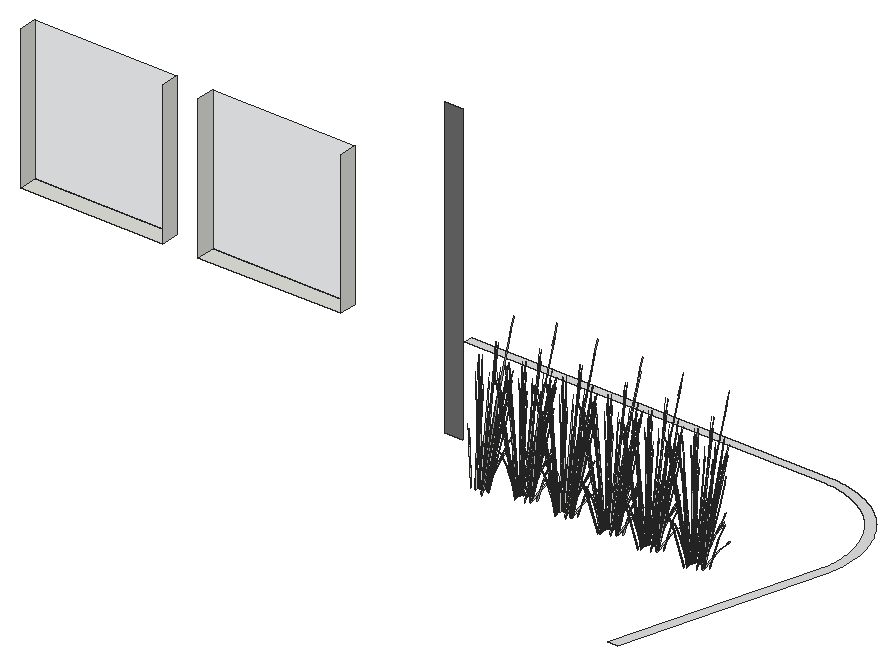
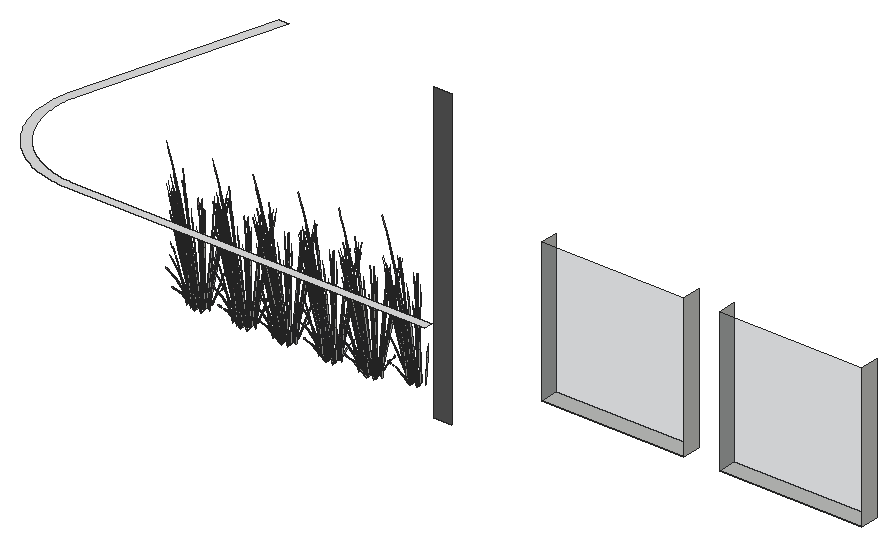
# SketchUp Ruby script. Lengths in inches.
U = 1.inch
M = Sketchup.active_model
def pt(a) = Geom::Point3d.new(a.map { |v| v * U })
def face(e, loops, mat)
  f = e.add_face(loops[0].map { |a| pt(a) })
  loops[1..].each { |l| e.add_face(l.map { |a| pt(a) }).erase! }
  f.material = f.back_material = mat if mat
  f
end
# faces: each face lists its corners as indices into pts; further lists are holes
def faces(e, pts, list, mat = nil) = list.each { |f| face(e, (f[0].is_a?(Array) ? f : [f]).map { |l| l.map { |i| pts[i] } }, mat) }
# xy, xz, yz: faces in a plane at the given z, y or x. An outline is a flat list of corners, or four numbers for a rectangle; further outlines are holes
def ring(l) = l.size == 4 ? [[l[0], l[1]], [l[2], l[1]], [l[2], l[3]], [l[0], l[3]]] : l.each_slice(2).to_a
def flat(e, list, mat, &to3) = list.each { |f| face(e, (f[0].is_a?(Array) ? f : [f]).map { |l| ring(l).map { |u, v| to3.(u, v) } }, mat) }
def xy(e, z, list, mat = nil) = flat(e, list, mat) { |x, y| [x, y, z] }
def xz(e, y, list, mat = nil) = flat(e, list, mat) { |x, z| [x, y, z] }
def yz(e, x, list, mat = nil) = flat(e, list, mat) { |y, z| [x, y, z] }
def lines(e, pts, list) = list.each { |a, b| e.add_line(pt(pts[a]), pt(pts[b])) }
# prism: a flat outline (further loops are holes) pulled along v
def prism(e, loops, v, mat = nil)
  f = face(e, loops, mat); d = Geom::Vector3d.new(v.map { |x| x * U })
  f.pushpull(f.normal.samedirection?(d) ? d.length : -d.length)
end
def box(e, o, s, mat = nil) = prism(e, [[o, [o[0] + s[0], o[1], o[2]], [o[0] + s[0], o[1] + s[1], o[2]], [o[0], o[1] + s[1], o[2]]]], [0, 0, s[2]], mat)
def at(x, y, z, deg = 0) = Geom::Transformation.translation(pt([x, y, z])) * Geom::Transformation.rotation(ORIGIN, Z_AXIS, deg.degrees)
def axes(o, x, y, z) = Geom::Transformation.new([*x, 0, *y, 0, *z, 0, *pt(o).to_a, 1])
def part(name) = M.definitions.add(name)
# library, detail: a bought-in or finely detailed component or shape, given as its bounding box
def library(name, o, s) = part(name).tap { |d| box(d.entities, o, s) }
def detail(e, o, s) = box(e.add_group.entities, o, s)
def put(e, d, t, mat = nil) = e.add_instance(d, t).tap { |i| i.material = mat if mat }
def group(e, t, mat = nil) = e.add_group.tap { |g| g.transformation = t; g.material = mat if mat }.entities
root = M.entities
M.materials.add("Glass_Basic_01").color = [105, 113, 122]
M.materials["Glass_Basic_01"].alpha = 0.25
M.materials.add("LightPink_Translucent").color = [144, 107, 117]
M.materials["LightPink_Translucent"].alpha = 0.75
M.materials.add("M01_Silver_Fog").color = [224, 224, 224]
M.materials.add("M06_Steel_Smoke").color = [114, 114, 114]
c1 = part("blade")
p = [[2.15,0.21,22],[0,0.17,0],[0.09,0.45,0],[2.18,0.31,22],[2.29,0.31,22],[0.38,0.45,0],
  [2.48,0.24,33],[2.49,0.24,33],[2.48,0.22,33]]
faces(c1.entities,p,[[0,1,2,3],[4,5,2,3],[6,3,4,7],[8,0,3,6]])
c2 = part("seeds")
p = [[0.3,-0.1,1.38],[-0.01,-0.03,1.59],[-0.01,-0.03,0.03],[0.14,-0.07,-0.07],[0.29,-0.03,3],[0.15,0.01,3.11]]
faces(c2.entities,p,[[0,1,2,3],[1,0,4,5]],"LightPink_Translucent")
c3 = part("blade with seeds")
put(c3.entities,c1,at(0,0,0))
put(c3.entities,c2,axes([2.4,0.25,30.99],[1.5799,-0.05474,1.17369],[-0.12525,1.92788,0.29478],[-0.07173,-0.02425,1.56792]))
xy(root,426,[[60,474,108,480],[120,474,168,480]])
xy(root,432,[[340.07,371.78,343.2,371.78,362.06,436.22,362.32,437.22,362.58,438.42,362.79,439.63,362.96,440.85,363.08,442.08,363.16,443.31,363.1875,444.54,363.17,445.77,363.1,447,362.99,448.22,362.83,449.44,362.63,450.66,362.38,451.86,362.08,453.06,361.74,454.24,361.35,455.41,360.92,456.5625,360.45,457.7,359.93,458.82,359.37,459.91,358.77,460.99,358.13,462.03,358.13,462.04,357.45,463.0625,356.73,464.0625,355.97,465.03,355.18,465.98,355.17,465.98,354.35,466.89,353.49,467.76,352.59,468.61,351.67,469.42,350.71,470.19,349.72,470.93,348.71,471.63,347.67,472.29,346.61,472.91,345.52,473.49,344.41,474.03,343.29,474.52,342.14,474.97,340.98,475.38,339.8,475.75,338.61,476.0625,337.41,476.34,336.2,476.5625,334.99,476.74,333.76,476.88,332.53,476.97,331.5,477,210,477,210,474,331.45,474,332.38,473.97,333.49,473.89,334.6,473.77,335.71,473.6,336.8,473.4,337.89,473.15,338.97,472.86,340.04,472.53,341.09,472.16,342.13,471.75,343.16,471.3,344.16,470.82,345.15,470.29,346.11,469.73,347.05,469.13,347.97,468.5,348.87,467.83,349.74,467.125,350.58,466.39,351.39,465.62,352.17,464.83,352.92,464,353.64,463.14,354.33,462.26,354.98,461.36,355.6,460.43,356.18,459.47,356.73,458.5,357.23,457.5,357.7,456.49,358.13,455.46,358.52,454.41,358.875,453.35,359.18,452.28,359.45,451.2,359.68,450.1,359.87,449,360.01,447.89,360.11,446.78,360.17,445.67,360.1875,444.55,360.16,443.43,360.09,442.32,359.98,441.21,359.83,440.1,359.63,439,359.4,437.91,359.17,437.01]],"M01_Silver_Fog")
xz(root,473,[[204,403,210,503]],"M06_Steel_Smoke")
xz(root,480,[[60,426,108,474],[120,426,168,474]],"Glass_Basic_01")
yz(root,60,[[474,426,480,474]])
yz(root,108,[[474,426,480,474]])
yz(root,120,[[474,426,480,474]])
yz(root,168,[[474,426,480,474]])
put(root,c3,axes([266.91,458.68,400.71],[0.03725,0.05374,1.77383],[-0.17957,0.48312,-0.16761],[-0.18186,0.0035,0.31391]))
put(root,c3,axes([280.52,458.68,400.71],[0.03725,0.05374,1.77383],[-0.17957,0.48312,-0.16761],[-0.18186,0.0035,0.31391]))
put(root,c3,axes([296.05,458.68,400.71],[0.03725,0.05374,1.77383],[-0.17957,0.48312,-0.16761],[-0.18186,0.0035,0.31391]))
put(root,c3,axes([238.73,459.53,401.05],[0.28589,0.33718,0.35414],[-0.32644,0.31919,-0.4572],[-0.16586,-0.04856,0.87481]))
put(root,c3,axes([252.44,459.53,401.05],[0.28589,0.33718,0.35414],[-0.32644,0.31919,-0.4572],[-0.16586,-0.04856,0.87481]))
put(root,c3,axes([267.69,459.53,401.05],[0.28589,0.33718,0.35414],[-0.32644,0.31919,-0.4572],[-0.16586,-0.04856,0.87481]))
put(root,c3,axes([281.3,459.53,401.05],[0.28589,0.33718,0.35414],[-0.32644,0.31919,-0.4572],[-0.16586,-0.04856,0.87481]))
put(root,c3,axes([296.83,459.53,401.05],[0.28589,0.33718,0.35414],[-0.32644,0.31919,-0.4572],[-0.16586,-0.04856,0.87481]))
put(root,c3,axes([227.09,457.28,401.05],[0.43736,-0.07697,0.35414],[0.11549,0.43998,-0.4572],[-0.12533,0.11818,0.87481]))
put(root,c3,axes([238.66,459.3125,401.03],[-0.0269,0.54769,-0.1216],[-0.50939,-0.01497,-0.67495],[-0.19618,-0.03804,1.02557]))
put(root,c3,axes([252.36,459.3125,401.03],[-0.0269,0.54769,-0.1216],[-0.50939,-0.01497,-0.67495],[-0.19618,-0.03804,1.02557]))
put(root,c3,axes([267.61,459.3125,401.03],[-0.0269,0.54769,-0.1216],[-0.50939,-0.01497,-0.67495],[-0.19618,-0.03804,1.02557]))
put(root,c3,axes([281.23,459.3125,401.03],[-0.0269,0.54769,-0.1216],[-0.50939,-0.01497,-0.67495],[-0.19618,-0.03804,1.02557]))
put(root,c3,axes([296.76,459.3125,401.03],[-0.0269,0.54769,-0.1216],[-0.50939,-0.01497,-0.67495],[-0.19618,-0.03804,1.02557]))
put(root,c3,axes([225.4,457.08,400.71],[0.06412,0.01444,1.77383],[0.19837,0.47583,-0.16761],[-0.13126,0.12489,0.31391]))
put(root,c3,axes([242.47,461.41,401.03],[-0.25281,-0.48765,-0.1216],[0.44869,-0.23964,-0.67495],[0.18908,-0.06434,1.02557]))
put(root,c3,axes([256.18,461.41,401.03],[-0.25281,-0.48765,-0.1216],[0.44869,-0.23964,-0.67495],[0.18908,-0.06434,1.02557]))
put(root,c3,axes([271.42,461.41,401.03],[-0.25281,-0.48765,-0.1216],[0.44869,-0.23964,-0.67495],[0.18908,-0.06434,1.02557]))
put(root,c3,axes([285.04,461.41,401.03],[-0.25281,-0.48765,-0.1216],[0.44869,-0.23964,-0.67495],[0.18908,-0.06434,1.02557]))
put(root,c3,axes([300.57,461.41,401.03],[-0.25281,-0.48765,-0.1216],[0.44869,-0.23964,-0.67495],[0.18908,-0.06434,1.02557]))
put(root,c3,axes([230.84,458.27,400.73],[-0.0253,0.40952,0.0643],[-0.38204,-0.01123,0.50621],[0.14634,0.04285,0.77189]))
put(root,c3,axes([230.87,458.14,400.73],[-0.37048,0.35486,0.48003],[-0.31952,-0.37685,0.3958],[0.17382,0.06546,0.9933]))
put(root,c3,axes([226.1,458.53,401.65],[0.44338,0.14375,-0.06488],[-0.13639,0.44245,-0.29416],[-0.07252,0.06718,0.97024]))
put(root,c3,axes([229.69,458.55,401.05],[-0.0776,-0.43378,0.35414],[0.44361,-0.11454,-0.4572],[0.11915,0.12431,0.87481]))
put(root,c3,axes([242.29,461.27,401.05],[-0.41757,-0.15024,0.35414],[0.12179,-0.4383,-0.4572],[0.16812,-0.04019,0.87481]))
put(root,c3,axes([256,461.27,401.05],[-0.41757,-0.15024,0.35414],[0.12179,-0.4383,-0.4572],[0.16812,-0.04019,0.87481]))
put(root,c3,axes([271.25,461.27,401.05],[-0.41757,-0.15024,0.35414],[0.12179,-0.4383,-0.4572],[0.16812,-0.04019,0.87481]))
put(root,c3,axes([284.86,461.27,401.05],[-0.41757,-0.15024,0.35414],[0.12179,-0.4383,-0.4572],[0.16812,-0.04019,0.87481]))
put(root,c3,axes([300.39,461.27,401.05],[-0.41757,-0.15024,0.35414],[0.12179,-0.4383,-0.4572],[0.16812,-0.04019,0.87481]))
put(root,c3,axes([229.99,456.06,400.47],[-0.43417,-0.27982,1.38283],[0.45844,-0.43566,0.59665],[0.14008,0.26255,1.33663]))
put(root,c3,axes([237.92,460.46,400.73],[0.14195,-0.49104,0.48003],[0.46669,0.16791,0.3958],[-0.18353,0.02951,0.9933]))
put(root,c3,axes([251.63,460.46,400.73],[0.14195,-0.49104,0.48003],[0.46669,0.16791,0.3958],[-0.18353,0.02951,0.9933]))
put(root,c3,axes([266.875,460.46,400.73],[0.14195,-0.49104,0.48003],[0.46669,0.16791,0.3958],[-0.18353,0.02951,0.9933]))
put(root,c3,axes([280.49,460.46,400.73],[0.14195,-0.49104,0.48003],[0.46669,0.16791,0.3958],[-0.18353,0.02951,0.9933]))
put(root,c3,axes([296.02,460.46,400.73],[0.14195,-0.49104,0.48003],[0.46669,0.16791,0.3958],[-0.18353,0.02951,0.9933]))
put(root,c3,axes([237.89,460.33,400.73],[-0.18454,-0.3672,0.0643],[0.33652,-0.17973,0.50621],[-0.14834,0.03546,0.77189]))
put(root,c3,axes([251.59,460.33,400.73],[-0.18454,-0.3672,0.0643],[0.33652,-0.17973,0.50621],[-0.14834,0.03546,0.77189]))
put(root,c3,axes([266.84,460.33,400.73],[-0.18454,-0.3672,0.0643],[0.33652,-0.17973,0.50621],[-0.14834,0.03546,0.77189]))
put(root,c3,axes([280.45,460.33,400.73],[-0.18454,-0.3672,0.0643],[0.33652,-0.17973,0.50621],[-0.14834,0.03546,0.77189]))
put(root,c3,axes([295.98,460.33,400.73],[-0.18454,-0.3672,0.0643],[0.33652,-0.17973,0.50621],[-0.14834,0.03546,0.77189]))
put(root,c3,axes([226.86,457.24,401.03],[0.46478,0.29695,-0.1216],[-0.26776,0.43004,-0.67495],[-0.13131,0.14949,1.02557]))
put(root,c3,axes([229.65,458.78,401.03],[0.2994,-0.46097,-0.1216],[0.43359,0.26557,-0.67495],[0.15072,0.13024,1.02557]))
put(root,c3,axes([227.68,458.15,401.05],[0.33997,-0.28354,0.35414],[0.32182,0.32376,-0.4572],[-0.04897,0.1645,0.87481]))
put(root,c3,axes([229.26,459.16,400.71],[0.00149,-0.0652,1.77383],[0.43058,-0.28766,-0.16761],[0.14956,0.10267,0.31391]))
put(root,c3,axes([227.37,458.41,400.73],[-0.4129,-0.02509,0.0643],[0.01132,-0.37891,0.50621],[-0.04321,0.14514,0.77189]))
put(root,c3,axes([227.5,458.45,400.73],[-0.35779,-0.36745,0.48003],[0.37996,-0.3169,0.3958],[-0.066,0.17239,0.9933]))
put(root,c3,axes([228.63,458.62,401.05],[0.15148,-0.41415,0.35414],[0.44193,0.12079,-0.4572],[0.04052,0.16674,0.87481]))
put(root,c3,axes([242.67,461.4,400.73],[0.18454,0.3672,0.0643],[-0.33652,0.17973,0.50621],[0.14834,-0.03546,0.77189]))
put(root,c3,axes([256.38,461.4,400.73],[0.18454,0.3672,0.0643],[-0.33652,0.17973,0.50621],[0.14834,-0.03546,0.77189]))
put(root,c3,axes([271.625,461.4,400.73],[0.18454,0.3672,0.0643],[-0.33652,0.17973,0.50621],[0.14834,-0.03546,0.77189]))
put(root,c3,axes([285.24,461.4,400.73],[0.18454,0.3672,0.0643],[-0.33652,0.17973,0.50621],[0.14834,-0.03546,0.77189]))
put(root,c3,axes([300.77,461.4,400.73],[0.18454,0.3672,0.0643],[-0.33652,0.17973,0.50621],[0.14834,-0.03546,0.77189]))
put(root,c3,axes([229.76,458.94,400.73],[-0.22836,0.34211,0.0643],[-0.3252,-0.19918,0.50621],[0.10513,0.10968,0.77189]))
put(root,c3,axes([242.64,461.27,400.73],[-0.14195,0.49104,0.48003],[-0.46669,-0.16791,0.3958],[0.18353,-0.02951,0.9933]))
put(root,c3,axes([256.34,461.27,400.73],[-0.14195,0.49104,0.48003],[-0.46669,-0.16791,0.3958],[0.18353,-0.02951,0.9933]))
put(root,c3,axes([271.59,461.27,400.73],[-0.14195,0.49104,0.48003],[-0.46669,-0.16791,0.3958],[0.18353,-0.02951,0.9933]))
put(root,c3,axes([285.2,461.27,400.73],[-0.14195,0.49104,0.48003],[-0.46669,-0.16791,0.3958],[0.18353,-0.02951,0.9933]))
put(root,c3,axes([300.73,461.27,400.73],[-0.14195,0.49104,0.48003],[-0.46669,-0.16791,0.3958],[0.18353,-0.02951,0.9933]))
put(root,c3,axes([229.23,460.1,401.65],[0.34721,-0.30895,-0.06488],[0.31814,0.33837,-0.29416],[0.0224,0.09588,0.97024]))
put(root,c3,axes([238.26,460.47,401.05],[0.41757,0.15024,0.35414],[-0.12179,0.4383,-0.4572],[-0.16812,0.04019,0.87481]))
put(root,c3,axes([251.97,460.47,401.05],[0.41757,0.15024,0.35414],[-0.12179,0.4383,-0.4572],[-0.16812,0.04019,0.87481]))
put(root,c3,axes([267.22,460.47,401.05],[0.41757,0.15024,0.35414],[-0.12179,0.4383,-0.4572],[-0.16812,0.04019,0.87481]))
put(root,c3,axes([280.83,460.47,401.05],[0.41757,0.15024,0.35414],[-0.12179,0.4383,-0.4572],[-0.16812,0.04019,0.87481]))
put(root,c3,axes([296.36,460.47,401.05],[0.41757,0.15024,0.35414],[-0.12179,0.4383,-0.4572],[-0.16812,0.04019,0.87481]))
put(root,c3,axes([229.86,458.85,400.73],[-0.49974,0.12359,0.48003],[-0.08673,-0.48481,0.3958],[0.11753,0.14288,0.9933]))
put(root,c3,axes([228.5,459,400.73],[-0.37023,0.18303,0.0643],[-0.18122,-0.33376,0.50621],[0.03575,0.14712,0.77189]))
put(root,c3,axes([226.33,458.47,400.72],[-0.01249,0.10657,1.74944],[0.35444,0.37075,-0.27667],[-0.09279,0.17532,0.14031]))
put(root,c3,axes([227.46,458.23,401.4],[0.55221,0.02668,-0.13498],[-0.01509,0.50521,-0.74919],[-0.03836,0.19458,1.13838]))
put(root,c3,axes([228.48,458.79,401.03],[0.49168,-0.25073,-0.1216],[0.24162,0.44501,-0.67495],[0.06487,0.18753,1.02557]))
put(root,c3,axes([228.625,458.96,401.0625],[-0.4951,-0.14079,0.53283],[0.1693,-0.46287,0.43934],[0.02975,0.18203,1.10256]))
put(root,c3,axes([243.47,462.86,400.71],[-0.04543,-0.04715,1.77383],[0.09938,-0.50538,-0.16761],[0.17896,-0.03229,0.31391]))
put(root,c3,axes([257.18,462.86,400.71],[-0.04543,-0.04715,1.77383],[0.09938,-0.50538,-0.16761],[0.17896,-0.03229,0.31391]))
put(root,c3,axes([272.43,462.86,400.71],[-0.04543,-0.04715,1.77383],[0.09938,-0.50538,-0.16761],[0.17896,-0.03229,0.31391]))
put(root,c3,axes([286.04,462.86,400.71],[-0.04543,-0.04715,1.77383],[0.09938,-0.50538,-0.16761],[0.17896,-0.03229,0.31391]))
put(root,c3,axes([301.57,462.86,400.71],[-0.04543,-0.04715,1.77383],[0.09938,-0.50538,-0.16761],[0.17896,-0.03229,0.31391]))
put(root,c3,axes([237.5625,460.8125,400.72],[-0.08205,0.06992,1.74944],[0.00698,0.51086,-0.27667],[-0.18807,0.06644,0.14031]))
put(root,c3,axes([251.27,460.8125,400.72],[-0.08205,0.06992,1.74944],[0.00698,0.51086,-0.27667],[-0.18807,0.06644,0.14031]))
put(root,c3,axes([266.52,460.8125,400.72],[-0.08205,0.06992,1.74944],[0.00698,0.51086,-0.27667],[-0.18807,0.06644,0.14031]))
put(root,c3,axes([280.13,460.8125,400.72],[-0.08205,0.06992,1.74944],[0.00698,0.51086,-0.27667],[-0.18807,0.06644,0.14031]))
put(root,c3,axes([295.66,460.8125,400.72],[-0.08205,0.06992,1.74944],[0.00698,0.51086,-0.27667],[-0.18807,0.06644,0.14031]))
put(root,c3,axes([238.09,460.32,401.03],[0.25281,0.48765,-0.1216],[-0.44869,0.23964,-0.67495],[-0.18908,0.06434,1.02557]))
put(root,c3,axes([251.8,460.32,401.03],[0.25281,0.48765,-0.1216],[-0.44869,0.23964,-0.67495],[-0.18908,0.06434,1.02557]))
put(root,c3,axes([267.04,460.32,401.03],[0.25281,0.48765,-0.1216],[-0.44869,0.23964,-0.67495],[-0.18908,0.06434,1.02557]))
put(root,c3,axes([280.66,460.32,401.03],[0.25281,0.48765,-0.1216],[-0.44869,0.23964,-0.67495],[-0.18908,0.06434,1.02557]))
put(root,c3,axes([296.1875,460.32,401.03],[0.25281,0.48765,-0.1216],[-0.44869,0.23964,-0.67495],[-0.18908,0.06434,1.02557]))
put(root,c3,axes([241.9,462.43,401.03],[0.0269,-0.54769,-0.1216],[0.50939,0.01497,-0.67495],[0.19618,0.03804,1.02557]))
put(root,c3,axes([255.61,462.43,401.03],[0.0269,-0.54769,-0.1216],[0.50939,0.01497,-0.67495],[0.19618,0.03804,1.02557]))
put(root,c3,axes([270.86,462.43,401.03],[0.0269,-0.54769,-0.1216],[0.50939,0.01497,-0.67495],[0.19618,0.03804,1.02557]))
put(root,c3,axes([284.47,462.43,401.03],[0.0269,-0.54769,-0.1216],[0.50939,0.01497,-0.67495],[0.19618,0.03804,1.02557]))
put(root,c3,axes([300,462.43,401.03],[0.0269,-0.54769,-0.1216],[0.50939,0.01497,-0.67495],[0.19618,0.03804,1.02557]))
put(root,c3,axes([241.82,462.21,401.05],[-0.28589,-0.33718,0.35414],[0.32644,-0.31919,-0.4572],[0.16586,0.04856,0.87481]))
put(root,c3,axes([255.53,462.21,401.05],[-0.28589,-0.33718,0.35414],[0.32644,-0.31919,-0.4572],[0.16586,0.04856,0.87481]))
put(root,c3,axes([270.78,462.21,401.05],[-0.28589,-0.33718,0.35414],[0.32644,-0.31919,-0.4572],[0.16586,0.04856,0.87481]))
put(root,c3,axes([284.39,462.21,401.05],[-0.28589,-0.33718,0.35414],[0.32644,-0.31919,-0.4572],[0.16586,0.04856,0.87481]))
put(root,c3,axes([299.92,462.21,401.05],[-0.28589,-0.33718,0.35414],[0.32644,-0.31919,-0.4572],[0.16586,0.04856,0.87481]))
put(root,c3,axes([226.29,459.5625,400.71],[0.057,-0.03251,1.77383],[0.47114,0.21627,-0.16761],[-0.01107,0.18007,0.31391]))
put(root,c3,axes([242.34,462.1,400.72],[0.10779,-0.00911,1.74944],[0.29564,-0.41839,-0.27667],[0.19172,0.05523,0.14031]))
put(root,c3,axes([256.05,462.1,400.72],[0.10779,-0.00911,1.74944],[0.29564,-0.41839,-0.27667],[0.19172,0.05523,0.14031]))
put(root,c3,axes([271.3,462.1,400.72],[0.10779,-0.00911,1.74944],[0.29564,-0.41839,-0.27667],[0.19172,0.05523,0.14031]))
put(root,c3,axes([284.91,462.1,400.72],[0.10779,-0.00911,1.74944],[0.29564,-0.41839,-0.27667],[0.19172,0.05523,0.14031]))
put(root,c3,axes([300.44,462.1,400.72],[0.10779,-0.00911,1.74944],[0.29564,-0.41839,-0.27667],[0.19172,0.05523,0.14031]))
put(root,c3,axes([238.03,461.6875,400.73],[-0.12461,-0.49565,0.48003],[0.48882,-0.08602,0.3958],[-0.14406,0.11657,0.9933]))
put(root,c3,axes([251.74,461.6875,400.73],[-0.12461,-0.49565,0.48003],[0.48882,-0.08602,0.3958],[-0.14406,0.11657,0.9933]))
put(root,c3,axes([266.99,461.6875,400.73],[-0.12461,-0.49565,0.48003],[0.48882,-0.08602,0.3958],[-0.14406,0.11657,0.9933]))
put(root,c3,axes([280.6,461.6875,400.73],[-0.12461,-0.49565,0.48003],[0.48882,-0.08602,0.3958],[-0.14406,0.11657,0.9933]))
put(root,c3,axes([296.13,461.6875,400.73],[-0.12461,-0.49565,0.48003],[0.48882,-0.08602,0.3958],[-0.14406,0.11657,0.9933]))
put(root,c3,axes([237.9375,461.59,400.73],[-0.34493,-0.22649,0.0643],[0.20082,-0.32253,0.50621],[-0.11059,0.10427,0.77189]))
put(root,c3,axes([251.64,461.59,400.73],[-0.34493,-0.22649,0.0643],[0.20082,-0.32253,0.50621],[-0.11059,0.10427,0.77189]))
put(root,c3,axes([266.89,461.59,400.73],[-0.34493,-0.22649,0.0643],[0.20082,-0.32253,0.50621],[-0.11059,0.10427,0.77189]))
put(root,c3,axes([280.51,461.59,400.73],[-0.34493,-0.22649,0.0643],[0.20082,-0.32253,0.50621],[-0.11059,0.10427,0.77189]))
put(root,c3,axes([296.04,461.59,400.73],[-0.34493,-0.22649,0.0643],[0.20082,-0.32253,0.50621],[-0.11059,0.10427,0.77189]))
put(root,c3,axes([228.37,459.79,400.72],[0.06369,0.08672,1.74944],[0.51399,0.03407,-0.27667],[0.05169,0.19126,0.14031]))
put(root,c3,axes([238.33,461.52,401.05],[0.43736,-0.07697,0.35414],[0.11549,0.43998,-0.4572],[-0.12533,0.11818,0.87481]))
put(root,c3,axes([252.04,461.52,401.05],[0.43736,-0.07697,0.35414],[0.11549,0.43998,-0.4572],[-0.12533,0.11818,0.87481]))
put(root,c3,axes([267.29,461.52,401.05],[0.43736,-0.07697,0.35414],[0.11549,0.43998,-0.4572],[-0.12533,0.11818,0.87481]))
put(root,c3,axes([280.9,461.52,401.05],[0.43736,-0.07697,0.35414],[0.11549,0.43998,-0.4572],[-0.12533,0.11818,0.87481]))
put(root,c3,axes([296.43,461.52,401.05],[0.43736,-0.07697,0.35414],[0.11549,0.43998,-0.4572],[-0.12533,0.11818,0.87481]))
put(root,c3,axes([236.65,461.33,400.71],[0.06412,0.01444,1.77383],[0.19837,0.47583,-0.16761],[-0.13126,0.12489,0.31391]))
put(root,c3,axes([250.36,461.33,400.71],[0.06412,0.01444,1.77383],[0.19837,0.47583,-0.16761],[-0.13126,0.12489,0.31391]))
put(root,c3,axes([265.6,461.33,400.71],[0.06412,0.01444,1.77383],[0.19837,0.47583,-0.16761],[-0.13126,0.12489,0.31391]))
put(root,c3,axes([279.22,461.33,400.71],[0.06412,0.01444,1.77383],[0.19837,0.47583,-0.16761],[-0.13126,0.12489,0.31391]))
put(root,c3,axes([294.75,461.33,400.71],[0.06412,0.01444,1.77383],[0.19837,0.47583,-0.16761],[-0.13126,0.12489,0.31391]))
put(root,c3,axes([242.08,462.52,400.73],[-0.0253,0.40952,0.0643],[-0.38204,-0.01123,0.50621],[0.14634,0.04285,0.77189]))
put(root,c3,axes([255.79,462.52,400.73],[-0.0253,0.40952,0.0643],[-0.38204,-0.01123,0.50621],[0.14634,0.04285,0.77189]))
put(root,c3,axes([271.04,462.52,400.73],[-0.0253,0.40952,0.0643],[-0.38204,-0.01123,0.50621],[0.14634,0.04285,0.77189]))
put(root,c3,axes([284.65,462.52,400.73],[-0.0253,0.40952,0.0643],[-0.38204,-0.01123,0.50621],[0.14634,0.04285,0.77189]))
put(root,c3,axes([300.18,462.52,400.73],[-0.0253,0.40952,0.0643],[-0.38204,-0.01123,0.50621],[0.14634,0.04285,0.77189]))
put(root,c3,axes([242.12,462.39,400.73],[-0.37048,0.35486,0.48003],[-0.31952,-0.37685,0.3958],[0.17382,0.06546,0.9933]))
put(root,c3,axes([255.82,462.39,400.73],[-0.37048,0.35486,0.48003],[-0.31952,-0.37685,0.3958],[0.17382,0.06546,0.9933]))
put(root,c3,axes([271.07,462.39,400.73],[-0.37048,0.35486,0.48003],[-0.31952,-0.37685,0.3958],[0.17382,0.06546,0.9933]))
put(root,c3,axes([284.69,462.39,400.73],[-0.37048,0.35486,0.48003],[-0.31952,-0.37685,0.3958],[0.17382,0.06546,0.9933]))
put(root,c3,axes([300.22,462.39,400.73],[-0.37048,0.35486,0.48003],[-0.31952,-0.37685,0.3958],[0.17382,0.06546,0.9933]))
put(root,c3,axes([237.34,462.77,401.65],[0.44338,0.14375,-0.06488],[-0.13639,0.44245,-0.29416],[-0.07252,0.06718,0.97024]))
put(root,c3,axes([251.05,462.77,401.65],[0.44338,0.14375,-0.06488],[-0.13639,0.44245,-0.29416],[-0.07252,0.06718,0.97024]))
put(root,c3,axes([266.3,462.77,401.65],[0.44338,0.14375,-0.06488],[-0.13639,0.44245,-0.29416],[-0.07252,0.06718,0.97024]))
put(root,c3,axes([279.91,462.77,401.65],[0.44338,0.14375,-0.06488],[-0.13639,0.44245,-0.29416],[-0.07252,0.06718,0.97024]))
put(root,c3,axes([295.44,462.77,401.65],[0.44338,0.14375,-0.06488],[-0.13639,0.44245,-0.29416],[-0.07252,0.06718,0.97024]))
put(root,c3,axes([240.9375,462.8,401.05],[-0.0776,-0.43378,0.35414],[0.44361,-0.11454,-0.4572],[0.11915,0.12431,0.87481]))
put(root,c3,axes([254.65,462.8,401.05],[-0.0776,-0.43378,0.35414],[0.44361,-0.11454,-0.4572],[0.11915,0.12431,0.87481]))
put(root,c3,axes([269.89,462.8,401.05],[-0.0776,-0.43378,0.35414],[0.44361,-0.11454,-0.4572],[0.11915,0.12431,0.87481]))
put(root,c3,axes([283.51,462.8,401.05],[-0.0776,-0.43378,0.35414],[0.44361,-0.11454,-0.4572],[0.11915,0.12431,0.87481]))
put(root,c3,axes([299.04,462.8,401.05],[-0.0776,-0.43378,0.35414],[0.44361,-0.11454,-0.4572],[0.11915,0.12431,0.87481]))
put(root,c3,axes([241.24,460.3,400.47],[-0.43417,-0.27982,1.38283],[0.45844,-0.43566,0.59665],[0.14008,0.26255,1.33663]))
put(root,c3,axes([254.94,460.3,400.47],[-0.43417,-0.27982,1.38283],[0.45844,-0.43566,0.59665],[0.14008,0.26255,1.33663]))
put(root,c3,axes([270.19,460.3,400.47],[-0.43417,-0.27982,1.38283],[0.45844,-0.43566,0.59665],[0.14008,0.26255,1.33663]))
put(root,c3,axes([283.81,460.3,400.47],[-0.43417,-0.27982,1.38283],[0.45844,-0.43566,0.59665],[0.14008,0.26255,1.33663]))
put(root,c3,axes([299.34,460.3,400.47],[-0.43417,-0.27982,1.38283],[0.45844,-0.43566,0.59665],[0.14008,0.26255,1.33663]))
put(root,c3,axes([238.11,461.48,401.03],[0.46478,0.29695,-0.1216],[-0.26776,0.43004,-0.67495],[-0.13131,0.14949,1.02557]))
put(root,c3,axes([251.81,461.48,401.03],[0.46478,0.29695,-0.1216],[-0.26776,0.43004,-0.67495],[-0.13131,0.14949,1.02557]))
put(root,c3,axes([267.0625,461.48,401.03],[0.46478,0.29695,-0.1216],[-0.26776,0.43004,-0.67495],[-0.13131,0.14949,1.02557]))
put(root,c3,axes([280.68,461.48,401.03],[0.46478,0.29695,-0.1216],[-0.26776,0.43004,-0.67495],[-0.13131,0.14949,1.02557]))
put(root,c3,axes([296.21,461.48,401.03],[0.46478,0.29695,-0.1216],[-0.26776,0.43004,-0.67495],[-0.13131,0.14949,1.02557]))
put(root,c3,axes([240.9,463.02,401.03],[0.2994,-0.46097,-0.1216],[0.43359,0.26557,-0.67495],[0.15072,0.13024,1.02557]))
put(root,c3,axes([254.61,463.02,401.03],[0.2994,-0.46097,-0.1216],[0.43359,0.26557,-0.67495],[0.15072,0.13024,1.02557]))
put(root,c3,axes([269.85,463.02,401.03],[0.2994,-0.46097,-0.1216],[0.43359,0.26557,-0.67495],[0.15072,0.13024,1.02557]))
put(root,c3,axes([283.47,463.02,401.03],[0.2994,-0.46097,-0.1216],[0.43359,0.26557,-0.67495],[0.15072,0.13024,1.02557]))
put(root,c3,axes([299,463.02,401.03],[0.2994,-0.46097,-0.1216],[0.43359,0.26557,-0.67495],[0.15072,0.13024,1.02557]))
put(root,c3,axes([238.92,462.4,401.05],[0.33997,-0.28354,0.35414],[0.32182,0.32376,-0.4572],[-0.04897,0.1645,0.87481]))
put(root,c3,axes([252.63,462.4,401.05],[0.33997,-0.28354,0.35414],[0.32182,0.32376,-0.4572],[-0.04897,0.1645,0.87481]))
put(root,c3,axes([267.88,462.4,401.05],[0.33997,-0.28354,0.35414],[0.32182,0.32376,-0.4572],[-0.04897,0.1645,0.87481]))
put(root,c3,axes([281.49,462.4,401.05],[0.33997,-0.28354,0.35414],[0.32182,0.32376,-0.4572],[-0.04897,0.1645,0.87481]))
put(root,c3,axes([297.02,462.4,401.05],[0.33997,-0.28354,0.35414],[0.32182,0.32376,-0.4572],[-0.04897,0.1645,0.87481]))
put(root,c3,axes([240.51,463.4,400.71],[0.00149,-0.0652,1.77383],[0.43058,-0.28766,-0.16761],[0.14956,0.10267,0.31391]))
put(root,c3,axes([254.21,463.4,400.71],[0.00149,-0.0652,1.77383],[0.43058,-0.28766,-0.16761],[0.14956,0.10267,0.31391]))
put(root,c3,axes([269.46,463.4,400.71],[0.00149,-0.0652,1.77383],[0.43058,-0.28766,-0.16761],[0.14956,0.10267,0.31391]))
put(root,c3,axes([283.08,463.4,400.71],[0.00149,-0.0652,1.77383],[0.43058,-0.28766,-0.16761],[0.14956,0.10267,0.31391]))
put(root,c3,axes([298.61,463.4,400.71],[0.00149,-0.0652,1.77383],[0.43058,-0.28766,-0.16761],[0.14956,0.10267,0.31391]))
put(root,c3,axes([238.62,462.66,400.73],[-0.4129,-0.02509,0.0643],[0.01132,-0.37891,0.50621],[-0.04321,0.14514,0.77189]))
put(root,c3,axes([252.32,462.66,400.73],[-0.4129,-0.02509,0.0643],[0.01132,-0.37891,0.50621],[-0.04321,0.14514,0.77189]))
put(root,c3,axes([267.57,462.66,400.73],[-0.4129,-0.02509,0.0643],[0.01132,-0.37891,0.50621],[-0.04321,0.14514,0.77189]))
put(root,c3,axes([281.19,462.66,400.73],[-0.4129,-0.02509,0.0643],[0.01132,-0.37891,0.50621],[-0.04321,0.14514,0.77189]))
put(root,c3,axes([296.72,462.66,400.73],[-0.4129,-0.02509,0.0643],[0.01132,-0.37891,0.50621],[-0.04321,0.14514,0.77189]))
put(root,c3,axes([238.75,462.69,400.73],[-0.35779,-0.36745,0.48003],[0.37996,-0.3169,0.3958],[-0.066,0.17239,0.9933]))
put(root,c3,axes([252.45,462.69,400.73],[-0.35779,-0.36745,0.48003],[0.37996,-0.3169,0.3958],[-0.066,0.17239,0.9933]))
put(root,c3,axes([267.7,462.69,400.73],[-0.35779,-0.36745,0.48003],[0.37996,-0.3169,0.3958],[-0.066,0.17239,0.9933]))
put(root,c3,axes([281.32,462.69,400.73],[-0.35779,-0.36745,0.48003],[0.37996,-0.3169,0.3958],[-0.066,0.17239,0.9933]))
put(root,c3,axes([296.85,462.69,400.73],[-0.35779,-0.36745,0.48003],[0.37996,-0.3169,0.3958],[-0.066,0.17239,0.9933]))
put(root,c3,axes([239.88,462.87,401.05],[0.15148,-0.41415,0.35414],[0.44193,0.12079,-0.4572],[0.04052,0.16674,0.87481]))
put(root,c3,axes([253.59,462.87,401.05],[0.15148,-0.41415,0.35414],[0.44193,0.12079,-0.4572],[0.04052,0.16674,0.87481]))
put(root,c3,axes([268.83,462.87,401.05],[0.15148,-0.41415,0.35414],[0.44193,0.12079,-0.4572],[0.04052,0.16674,0.87481]))
put(root,c3,axes([282.45,462.87,401.05],[0.15148,-0.41415,0.35414],[0.44193,0.12079,-0.4572],[0.04052,0.16674,0.87481]))
put(root,c3,axes([297.98,462.87,401.05],[0.15148,-0.41415,0.35414],[0.44193,0.12079,-0.4572],[0.04052,0.16674,0.87481]))
put(root,c3,axes([241.01,463.19,400.73],[-0.22836,0.34211,0.0643],[-0.3252,-0.19918,0.50621],[0.10513,0.10968,0.77189]))
put(root,c3,axes([254.72,463.19,400.73],[-0.22836,0.34211,0.0643],[-0.3252,-0.19918,0.50621],[0.10513,0.10968,0.77189]))
put(root,c3,axes([269.96,463.19,400.73],[-0.22836,0.34211,0.0643],[-0.3252,-0.19918,0.50621],[0.10513,0.10968,0.77189]))
put(root,c3,axes([283.58,463.19,400.73],[-0.22836,0.34211,0.0643],[-0.3252,-0.19918,0.50621],[0.10513,0.10968,0.77189]))
put(root,c3,axes([299.11,463.19,400.73],[-0.22836,0.34211,0.0643],[-0.3252,-0.19918,0.50621],[0.10513,0.10968,0.77189]))
put(root,c3,axes([240.47,464.34,401.65],[0.34721,-0.30895,-0.06488],[0.31814,0.33837,-0.29416],[0.0224,0.09588,0.97024]))
put(root,c3,axes([254.18,464.34,401.65],[0.34721,-0.30895,-0.06488],[0.31814,0.33837,-0.29416],[0.0224,0.09588,0.97024]))
put(root,c3,axes([269.43,464.34,401.65],[0.34721,-0.30895,-0.06488],[0.31814,0.33837,-0.29416],[0.0224,0.09588,0.97024]))
put(root,c3,axes([283.04,464.34,401.65],[0.34721,-0.30895,-0.06488],[0.31814,0.33837,-0.29416],[0.0224,0.09588,0.97024]))
put(root,c3,axes([298.57,464.34,401.65],[0.34721,-0.30895,-0.06488],[0.31814,0.33837,-0.29416],[0.0224,0.09588,0.97024]))
put(root,c3,axes([241.1,463.09,400.73],[-0.49974,0.12359,0.48003],[-0.08673,-0.48481,0.3958],[0.11753,0.14288,0.9933]))
put(root,c3,axes([254.8125,463.09,400.73],[-0.49974,0.12359,0.48003],[-0.08673,-0.48481,0.3958],[0.11753,0.14288,0.9933]))
put(root,c3,axes([270.06,463.09,400.73],[-0.49974,0.12359,0.48003],[-0.08673,-0.48481,0.3958],[0.11753,0.14288,0.9933]))
put(root,c3,axes([283.67,463.09,400.73],[-0.49974,0.12359,0.48003],[-0.08673,-0.48481,0.3958],[0.11753,0.14288,0.9933]))
put(root,c3,axes([299.2,463.09,400.73],[-0.49974,0.12359,0.48003],[-0.08673,-0.48481,0.3958],[0.11753,0.14288,0.9933]))
put(root,c3,axes([239.74,463.24,400.73],[-0.37023,0.18303,0.0643],[-0.18122,-0.33376,0.50621],[0.03575,0.14712,0.77189]))
put(root,c3,axes([253.45,463.24,400.73],[-0.37023,0.18303,0.0643],[-0.18122,-0.33376,0.50621],[0.03575,0.14712,0.77189]))
put(root,c3,axes([268.7,463.24,400.73],[-0.37023,0.18303,0.0643],[-0.18122,-0.33376,0.50621],[0.03575,0.14712,0.77189]))
put(root,c3,axes([282.31,463.24,400.73],[-0.37023,0.18303,0.0643],[-0.18122,-0.33376,0.50621],[0.03575,0.14712,0.77189]))
put(root,c3,axes([297.84,463.24,400.73],[-0.37023,0.18303,0.0643],[-0.18122,-0.33376,0.50621],[0.03575,0.14712,0.77189]))
put(root,c3,axes([237.57,462.72,400.72],[-0.01249,0.10657,1.74944],[0.35444,0.37075,-0.27667],[-0.09279,0.17532,0.14031]))
put(root,c3,axes([251.28,462.72,400.72],[-0.01249,0.10657,1.74944],[0.35444,0.37075,-0.27667],[-0.09279,0.17532,0.14031]))
put(root,c3,axes([266.53,462.72,400.72],[-0.01249,0.10657,1.74944],[0.35444,0.37075,-0.27667],[-0.09279,0.17532,0.14031]))
put(root,c3,axes([280.14,462.72,400.72],[-0.01249,0.10657,1.74944],[0.35444,0.37075,-0.27667],[-0.09279,0.17532,0.14031]))
put(root,c3,axes([295.67,462.72,400.72],[-0.01249,0.10657,1.74944],[0.35444,0.37075,-0.27667],[-0.09279,0.17532,0.14031]))
put(root,c3,axes([238.71,462.48,401.4],[0.55221,0.02668,-0.13498],[-0.01509,0.50521,-0.74919],[-0.03836,0.19458,1.13838]))
put(root,c3,axes([252.42,462.48,401.4],[0.55221,0.02668,-0.13498],[-0.01509,0.50521,-0.74919],[-0.03836,0.19458,1.13838]))
put(root,c3,axes([267.66,462.48,401.4],[0.55221,0.02668,-0.13498],[-0.01509,0.50521,-0.74919],[-0.03836,0.19458,1.13838]))
put(root,c3,axes([281.28,462.48,401.4],[0.55221,0.02668,-0.13498],[-0.01509,0.50521,-0.74919],[-0.03836,0.19458,1.13838]))
put(root,c3,axes([296.81,462.48,401.4],[0.55221,0.02668,-0.13498],[-0.01509,0.50521,-0.74919],[-0.03836,0.19458,1.13838]))
put(root,c3,axes([239.73,463.04,401.03],[0.49168,-0.25073,-0.1216],[0.24162,0.44501,-0.67495],[0.06487,0.18753,1.02557]))
put(root,c3,axes([253.4375,463.04,401.03],[0.49168,-0.25073,-0.1216],[0.24162,0.44501,-0.67495],[0.06487,0.18753,1.02557]))
put(root,c3,axes([268.69,463.04,401.03],[0.49168,-0.25073,-0.1216],[0.24162,0.44501,-0.67495],[0.06487,0.18753,1.02557]))
put(root,c3,axes([282.3,463.04,401.03],[0.49168,-0.25073,-0.1216],[0.24162,0.44501,-0.67495],[0.06487,0.18753,1.02557]))
put(root,c3,axes([297.83,463.04,401.03],[0.49168,-0.25073,-0.1216],[0.24162,0.44501,-0.67495],[0.06487,0.18753,1.02557]))
put(root,c3,axes([239.87,463.21,401.0625],[-0.4951,-0.14079,0.53283],[0.1693,-0.46287,0.43934],[0.02975,0.18203,1.10256]))
put(root,c3,axes([253.58,463.21,401.0625],[-0.4951,-0.14079,0.53283],[0.1693,-0.46287,0.43934],[0.02975,0.18203,1.10256]))
put(root,c3,axes([268.83,463.21,401.0625],[-0.4951,-0.14079,0.53283],[0.1693,-0.46287,0.43934],[0.02975,0.18203,1.10256]))
put(root,c3,axes([282.44,463.21,401.0625],[-0.4951,-0.14079,0.53283],[0.1693,-0.46287,0.43934],[0.02975,0.18203,1.10256]))
put(root,c3,axes([297.97,463.21,401.0625],[-0.4951,-0.14079,0.53283],[0.1693,-0.46287,0.43934],[0.02975,0.18203,1.10256]))
put(root,c3,axes([237.53,463.8125,400.71],[0.057,-0.03251,1.77383],[0.47114,0.21627,-0.16761],[-0.01107,0.18007,0.31391]))
put(root,c3,axes([251.24,463.8125,400.71],[0.057,-0.03251,1.77383],[0.47114,0.21627,-0.16761],[-0.01107,0.18007,0.31391]))
put(root,c3,axes([266.49,463.8125,400.71],[0.057,-0.03251,1.77383],[0.47114,0.21627,-0.16761],[-0.01107,0.18007,0.31391]))
put(root,c3,axes([280.1,463.8125,400.71],[0.057,-0.03251,1.77383],[0.47114,0.21627,-0.16761],[-0.01107,0.18007,0.31391]))
put(root,c3,axes([295.63,463.8125,400.71],[0.057,-0.03251,1.77383],[0.47114,0.21627,-0.16761],[-0.01107,0.18007,0.31391]))
put(root,c3,axes([239.61,464.04,400.72],[0.06369,0.08672,1.74944],[0.51399,0.03407,-0.27667],[0.05169,0.19126,0.14031]))
put(root,c3,axes([253.32,464.04,400.72],[0.06369,0.08672,1.74944],[0.51399,0.03407,-0.27667],[0.05169,0.19126,0.14031]))
put(root,c3,axes([268.57,464.04,400.72],[0.06369,0.08672,1.74944],[0.51399,0.03407,-0.27667],[0.05169,0.19126,0.14031]))
put(root,c3,axes([282.18,464.04,400.72],[0.06369,0.08672,1.74944],[0.51399,0.03407,-0.27667],[0.05169,0.19126,0.14031]))
put(root,c3,axes([297.71,464.04,400.72],[0.06369,0.08672,1.74944],[0.51399,0.03407,-0.27667],[0.05169,0.19126,0.14031]))
